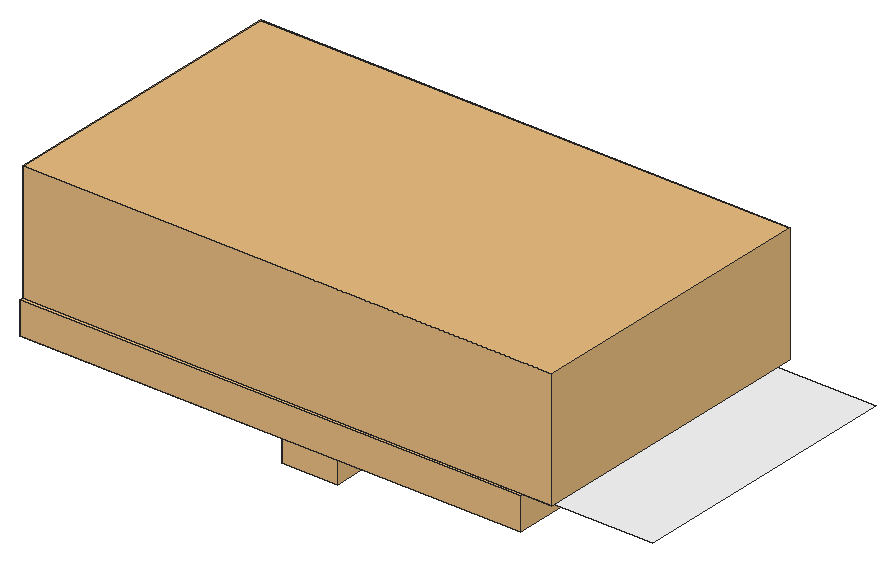
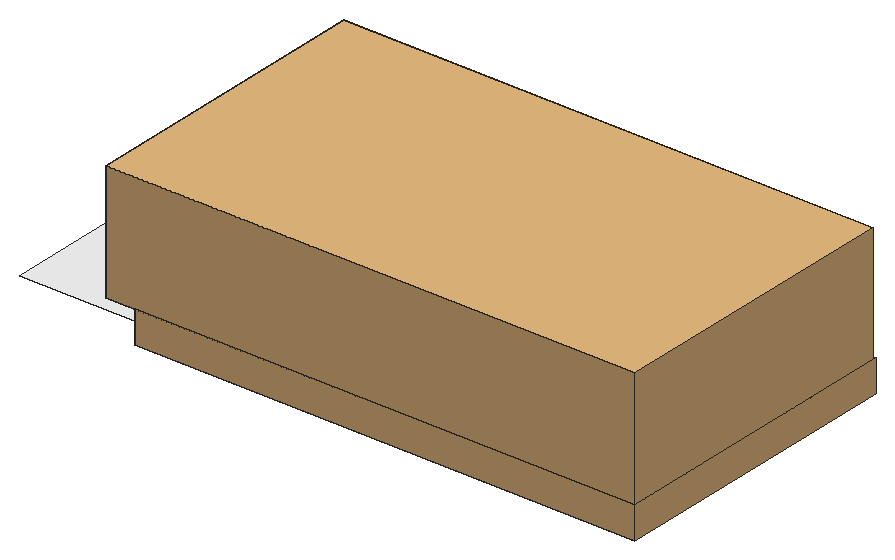
# SketchUp Ruby script. Lengths in inches.
U = 1.inch
M = Sketchup.active_model
def pt(a) = Geom::Point3d.new(a.map { |v| v * U })
def face(e, loops, mat)
  f = e.add_face(loops[0].map { |a| pt(a) })
  loops[1..].each { |l| e.add_face(l.map { |a| pt(a) }).erase! }
  f.material = f.back_material = mat if mat
  f
end
# faces: each face lists its corners as indices into pts; further lists are holes
def faces(e, pts, list, mat = nil) = list.each { |f| face(e, (f[0].is_a?(Array) ? f : [f]).map { |l| l.map { |i| pts[i] } }, mat) }
# xy, xz, yz: faces in a plane at the given z, y or x. An outline is a flat list of corners, or four numbers for a rectangle; further outlines are holes
def ring(l) = l.size == 4 ? [[l[0], l[1]], [l[2], l[1]], [l[2], l[3]], [l[0], l[3]]] : l.each_slice(2).to_a
def flat(e, list, mat, &to3) = list.each { |f| face(e, (f[0].is_a?(Array) ? f : [f]).map { |l| ring(l).map { |u, v| to3.(u, v) } }, mat) }
def xy(e, z, list, mat = nil) = flat(e, list, mat) { |x, y| [x, y, z] }
def xz(e, y, list, mat = nil) = flat(e, list, mat) { |x, z| [x, y, z] }
def yz(e, x, list, mat = nil) = flat(e, list, mat) { |y, z| [x, y, z] }
def lines(e, pts, list) = list.each { |a, b| e.add_line(pt(pts[a]), pt(pts[b])) }
# prism: a flat outline (further loops are holes) pulled along v
def prism(e, loops, v, mat = nil)
  f = face(e, loops, mat); d = Geom::Vector3d.new(v.map { |x| x * U })
  f.pushpull(f.normal.samedirection?(d) ? d.length : -d.length)
end
def box(e, o, s, mat = nil) = prism(e, [[o, [o[0] + s[0], o[1], o[2]], [o[0] + s[0], o[1] + s[1], o[2]], [o[0], o[1] + s[1], o[2]]]], [0, 0, s[2]], mat)
def at(x, y, z, deg = 0) = Geom::Transformation.translation(pt([x, y, z])) * Geom::Transformation.rotation(ORIGIN, Z_AXIS, deg.degrees)
def axes(o, x, y, z) = Geom::Transformation.new([*x, 0, *y, 0, *z, 0, *pt(o).to_a, 1])
def part(name) = M.definitions.add(name)
# library, detail: a bought-in or finely detailed component or shape, given as its bounding box
def library(name, o, s) = part(name).tap { |d| box(d.entities, o, s) }
def detail(e, o, s) = box(e.add_group.entities, o, s)
def put(e, d, t, mat = nil) = e.add_instance(d, t).tap { |i| i.material = mat if mat }
def group(e, t, mat = nil) = e.add_group.tap { |g| g.transformation = t; g.material = mat if mat }.entities
root = M.entities
M.materials.add("1421 AP 8232 ELEGANT GREY").color = [96, 96, 96]
M.materials.add("[Metal Seamed]").color = [36, 36, 35]
M.materials.add("[Quartz Light Grey]").color = [251, 251, 252]
c1 = library("Group\#16",[0,0,0],[139.79,84,8.95])
c2 = library("5",[-6.25,-6.25,-13.16],[15.58,15.58,13.16])
c3 = library("Group\#18",[0,-2,0],[147.82,83,33.01])
xy(root,119.5,[[115.18,204,114.86,204.04,114.79,204.05,114.71,204.07,114.63,204.08,114.56,204.1,114.48,204.125,114.41,204.15,114.33,204.17,114.19,204.23,114.11,204.26,114.04,204.29,113.97,204.33,113.9,204.36,113.83,204.4,113.77,204.44,113.7,204.48,113.63,204.53,113.57,204.57,113.45,204.67,113.38,204.72,113.33,204.77,113.27,204.82,113.1,204.99,112.95,205.17,112.91,205.24,112.86,205.3,112.82,205.37,112.78,205.43,112.66,205.64,112.59,205.78,112.5625,205.85,112.53,205.92,112.51,206,112.48,206.07,112.46,206.15,112.4375,206.22,112.42,206.3,112.38,206.45,112.36,206.61,112.35,206.6875,112.34,206.76,112.34,206.84,112.33,206.92,112.33,207.08,112.34,207.16,112.34,207.24,112.35,207.3125,112.36,207.39,112.38,207.55,112.42,207.7,112.4375,207.78,112.46,207.85,112.48,207.93,112.51,208,112.53,208.08,112.5625,208.15,112.59,208.22,112.66,208.36,112.78,208.57,112.82,208.63,112.86,208.7,112.91,208.76,112.95,208.83,113.1,209.01,113.27,209.18,113.33,209.23,113.38,209.28,113.45,209.33,113.57,209.43,113.63,209.47,113.7,209.52,113.77,209.56,113.83,209.6,113.9,209.64,113.97,209.67,114.04,209.71,114.11,209.74,114.19,209.77,114.33,209.83,114.41,209.85,114.48,209.875,114.56,209.9,114.63,209.92,114.71,209.93,114.79,209.95,114.86,209.96,115.18,210,115.49,210,115.65,209.98,115.72,209.97,115.88,209.95,115.96,209.93,116.03,209.92,116.11,209.9,116.19,209.875,116.26,209.85,116.33,209.83,116.41,209.8,116.55,209.74,116.625,209.71,116.7,209.67,116.76,209.64,116.97,209.52,117.03,209.47,117.1,209.43,117.4,209.18,117.45,209.12,117.51,209.07,117.5625,209.01,117.61,208.95,117.71,208.83,117.76,208.76,117.81,208.7,117.85,208.63,117.89,208.57,118.01,208.36,118.13,208.08,118.16,208,118.1875,207.93,118.21,207.85,118.23,207.78,118.25,207.7,118.27,207.625,118.28,207.55,118.3,207.47,118.31,207.39,118.32,207.3125,118.32,207.24,118.33,207.16,118.33,206.84,118.32,206.76,118.32,206.6875,118.31,206.61,118.3,206.53,118.28,206.45,118.27,206.375,118.25,206.3,118.23,206.22,118.21,206.15,118.1875,206.07,118.16,206,118.13,205.92,118.01,205.64,117.89,205.43,117.85,205.37,117.81,205.3,117.76,205.24,117.71,205.17,117.61,205.05,117.5625,204.99,117.51,204.93,117.45,204.88,117.4,204.82,117.1,204.57,117.03,204.53,116.97,204.48,116.76,204.36,116.7,204.33,116.625,204.29,116.55,204.26,116.41,204.2,116.33,204.17,116.26,204.15,116.19,204.125,116.11,204.1,116.03,204.08,115.96,204.07,115.88,204.05,115.72,204.03,115.65,204.02,115.49,204]],"[Quartz Light Grey]")
xy(root,126,[[60,187,174,187,174,193,216,193,216,271,60,271]],"[Quartz Light Grey]")
xz(root,204,[[115.18,117,115.25,119.5],[115.25,117,115.33,119.5],[115.33,117,115.41,119.5],[115.41,117,115.49,119.5]],"[Quartz Light Grey]")
xz(root,210,[[115.18,117,115.25,119.5],[115.25,117,115.33,119.5],[115.33,117,115.41,119.5],[115.41,117,115.49,119.5]],"[Quartz Light Grey]")
yz(root,72,[[206.84,117,206.92,119.5],[206.92,117,207,119.5],[207,117,207.08,119.5],[207.08,117,207.16,119.5]],"[Quartz Light Grey]")
yz(root,112.33,[[206.92,117,207,119.5],[207,117,207.08,119.5]],"[Quartz Light Grey]")
yz(root,112.34,[[206.76,117,206.84,119.5],[207.16,117,207.24,119.5]],"[Quartz Light Grey]")
yz(root,118.32,[[206.6875,117,206.76,119.5],[207.24,117,207.3125,119.5]],"[Quartz Light Grey]")
yz(root,118.33,[[206.84,117,206.92,119.5],[206.92,117,207,119.5],[207,117,207.08,119.5],[207.08,117,207.16,119.5]],"[Quartz Light Grey]")
yz(root,158.67,[[206.84,117,206.92,119.5],[206.92,117,207,119.5],[207,117,207.08,119.5],[207.08,117,207.16,119.5]],"[Quartz Light Grey]")
yz(root,158.68,[[206.6875,117,206.76,119.5],[207.24,117,207.3125,119.5]],"[Quartz Light Grey]")
p = [[114.86,204.04,117],[114.79,204.05,117],[114.79,204.05,119.5],[114.86,204.04,119.5],[114.94,204.03,117],[114.94,204.03,119.5],
  [115.02,204.02,117],[115.02,204.02,119.5],[115.1,204.01,117],[115.1,204.01,119.5],[115.18,204,117],[115.18,204,119.5],
  [115.57,204.01,117],[115.49,204,117],[115.49,204,119.5],[115.57,204.01,119.5],[115.65,204.02,117],[115.65,204.02,119.5],
  [115.72,204.03,117],[115.72,204.03,119.5],[115.8,204.04,117],[115.8,204.04,119.5],[115.88,204.05,117],[115.88,204.05,119.5],
  [69.78,204.1,117],[69.7,204.08,117],[69.7,204.08,119.5],[69.78,204.1,119.5],[69.85,204.125,117],[69.85,204.125,119.5],
  [69.93,204.15,117],[69.93,204.15,119.5],[70,204.17,117],[70,204.17,119.5],[114.41,204.15,117],[114.33,204.17,117],
  [114.33,204.17,119.5],[114.41,204.15,119.5],[114.48,204.125,117],[114.48,204.125,119.5],[114.56,204.1,117],[114.56,204.1,119.5],
  [114.63,204.08,117],[114.63,204.08,119.5],[114.71,204.07,117],[114.71,204.07,119.5],[115.96,204.07,117],[115.96,204.07,119.5],
  [116.03,204.08,117],[116.03,204.08,119.5],[116.11,204.1,117],[116.11,204.1,119.5],[116.19,204.125,117],[116.19,204.125,119.5],
  [116.26,204.15,117],[116.26,204.15,119.5],[116.33,204.17,117],[116.33,204.17,119.5],[70.08,204.2,117],[70.08,204.2,119.5],
  [70.15,204.23,117],[70.15,204.23,119.5],[70.22,204.26,117],[70.22,204.26,119.5],[114.19,204.23,117],[114.11,204.26,117],
  [114.11,204.26,119.5],[114.19,204.23,119.5],[114.26,204.2,117],[114.26,204.2,119.5],[116.41,204.2,117],[116.41,204.2,119.5],
  [116.48,204.23,117],[116.48,204.23,119.5],[116.55,204.26,117],[116.55,204.26,119.5],[70.29,204.29,117],[70.29,204.29,119.5],
  [70.36,204.33,117],[70.36,204.33,119.5],[70.43,204.36,117],[70.43,204.36,119.5],[113.97,204.33,117],[113.9,204.36,117],
  [113.9,204.36,119.5],[113.97,204.33,119.5],[114.04,204.29,117],[114.04,204.29,119.5],[116.625,204.29,117],[116.625,204.29,119.5],
  [116.7,204.33,117],[116.7,204.33,119.5],[116.76,204.36,117],[116.76,204.36,119.5],[70.5,204.4,117],[70.5,204.4,119.5],
  [70.57,204.44,117],[70.57,204.44,119.5],[70.63,204.48,117],[70.63,204.48,119.5],[113.77,204.44,117],[113.7,204.48,117],
  [113.7,204.48,119.5],[113.77,204.44,119.5],[113.83,204.4,117],[113.83,204.4,119.5],[116.83,204.4,117],[116.83,204.4,119.5],
  [116.9,204.44,117],[116.9,204.44,119.5],[116.97,204.48,117],[116.97,204.48,119.5],[70.7,204.53,117],[70.7,204.53,119.5],
  [70.76,204.57,117],[70.76,204.57,119.5],[113.63,204.53,117],[113.57,204.57,117],[113.57,204.57,119.5],[113.63,204.53,119.5],
  [117.03,204.53,117],[117.03,204.53,119.5],[117.1,204.57,117],[117.1,204.57,119.5],[70.83,204.62,117],[70.83,204.62,119.5],
  [70.89,204.67,117],[70.89,204.67,119.5],[113.51,204.62,117],[113.45,204.67,117],[113.45,204.67,119.5],[113.51,204.62,119.5],
  [117.16,204.62,117],[117.16,204.62,119.5],[117.22,204.67,117],[117.22,204.67,119.5],[70.95,204.72,117],[70.95,204.72,119.5],
  [71.01,204.77,117],[71.01,204.77,119.5],[113.38,204.72,117],[113.33,204.77,117],[113.33,204.77,119.5],[113.38,204.72,119.5],
  [117.28,204.72,117],[117.28,204.72,119.5],[117.34,204.77,117],[117.34,204.77,119.5],[71.07,204.82,117],[71.07,204.82,119.5],
  [71.12,204.88,117],[71.12,204.88,119.5],[113.27,204.82,117],[113.21,204.88,117],[113.21,204.88,119.5],[113.27,204.82,119.5],
  [117.4,204.82,117],[117.4,204.82,119.5],[117.45,204.88,117],[117.45,204.88,119.5],[71.18,204.93,117],[71.18,204.93,119.5],
  [71.23,204.99,117],[71.23,204.99,119.5],[113.16,204.93,117],[113.1,204.99,117],[113.1,204.99,119.5],[113.16,204.93,119.5],
  [117.51,204.93,117],[117.51,204.93,119.5],[117.5625,204.99,117],[117.5625,204.99,119.5],[71.28,205.05,117],[71.28,205.05,119.5],
  [113.05,205.05,117],[113.05,205.05,119.5],[117.61,205.05,117],[117.61,205.05,119.5],[71.33,205.11,117],[71.33,205.11,119.5],
  [71.38,205.17,117],[71.38,205.17,119.5],[113,205.11,117],[112.95,205.17,117],[112.95,205.17,119.5],[113,205.11,119.5],
  [117.66,205.11,117],[117.66,205.11,119.5],[117.71,205.17,117],[117.71,205.17,119.5],[159.34,205.11,117],[159.29,205.17,117],
  [159.29,205.17,119.5],[159.34,205.11,119.5],[71.43,205.24,117],[71.43,205.24,119.5],[71.47,205.3,117],[71.47,205.3,119.5],
  [112.91,205.24,117],[112.86,205.3,117],[112.86,205.3,119.5],[112.91,205.24,119.5],[117.76,205.24,117],[117.76,205.24,119.5],
  [117.81,205.3,117],[117.81,205.3,119.5],[159.24,205.24,117],[159.19,205.3,117],[159.19,205.3,119.5],[159.24,205.24,119.5],
  [71.52,205.37,117],[71.52,205.37,119.5],[112.82,205.37,117],[112.82,205.37,119.5],[117.85,205.37,117],[117.85,205.37,119.5],
  [159.15,205.37,117],[159.15,205.37,119.5],[71.56,205.43,117],[71.56,205.43,119.5],[71.6,205.5,117],[71.6,205.5,119.5],
  [112.78,205.43,117],[112.74,205.5,117],[112.74,205.5,119.5],[112.78,205.43,119.5],[117.89,205.43,117],[117.89,205.43,119.5],
  [117.93,205.5,117],[117.93,205.5,119.5],[159.11,205.43,117],[159.07,205.5,117],[159.07,205.5,119.5],[159.11,205.43,119.5],
  [71.64,205.57,117],[71.64,205.57,119.5],[112.7,205.57,117],[112.7,205.57,119.5],[117.97,205.57,117],[117.97,205.57,119.5],
  [159.03,205.57,117],[159.03,205.57,119.5],[71.67,205.64,117],[71.67,205.64,119.5],[71.71,205.71,117],[71.71,205.71,119.5],
  [112.66,205.64,117],[112.625,205.71,117],[112.625,205.71,119.5],[112.66,205.64,119.5],[118.01,205.64,117],[118.01,205.64,119.5],
  [118.04,205.71,117],[118.04,205.71,119.5],[158.99,205.64,117],[158.96,205.71,117],[158.96,205.71,119.5],[158.99,205.64,119.5],
  [71.74,205.78,117],[71.74,205.78,119.5],[112.59,205.78,117],[112.59,205.78,119.5],[118.07,205.78,117],[118.07,205.78,119.5],
  [158.93,205.78,117],[158.93,205.78,119.5],[71.77,205.85,117],[71.77,205.85,119.5],[112.5625,205.85,117],[112.5625,205.85,119.5],
  [118.1,205.85,117],[118.1,205.85,119.5],[158.9,205.85,117],[158.9,205.85,119.5],[71.8,205.92,117],[71.8,205.92,119.5],
  [71.83,206,117],[71.83,206,119.5],[112.53,205.92,117],[112.51,206,117],[112.51,206,119.5],[112.53,205.92,119.5],
  [118.13,205.92,117],[118.13,205.92,119.5],[118.16,206,117],[118.16,206,119.5],[158.87,205.92,117],[158.84,206,117],
  [158.84,206,119.5],[158.87,205.92,119.5],[71.85,206.07,117],[71.85,206.07,119.5],[112.48,206.07,117],[112.48,206.07,119.5],
  [118.1875,206.07,117],[118.1875,206.07,119.5],[158.8125,206.07,117],[158.8125,206.07,119.5],[71.875,206.15,117],[71.875,206.15,119.5],
  [71.9,206.22,117],[71.9,206.22,119.5],[112.46,206.15,117],[112.4375,206.22,117],[112.4375,206.22,119.5],[112.46,206.15,119.5],
  [118.21,206.15,117],[118.21,206.15,119.5],[118.23,206.22,117],[118.23,206.22,119.5],[158.79,206.15,117],[158.77,206.22,117],
  [158.77,206.22,119.5],[158.79,206.15,119.5],[71.92,206.3,117],[71.92,206.3,119.5],[112.42,206.3,117],[112.42,206.3,119.5],
  [118.25,206.3,117],[118.25,206.3,119.5],[158.75,206.3,117],[158.75,206.3,119.5],[71.93,206.375,117],[71.93,206.375,119.5],
  [112.4,206.375,117],[112.4,206.375,119.5],[118.27,206.375,117],[118.27,206.375,119.5],[158.73,206.375,117],[158.73,206.375,119.5],
  [71.95,206.45,117],[71.95,206.45,119.5],[112.38,206.45,117],[112.38,206.45,119.5],[118.28,206.45,117],[118.28,206.45,119.5],
  [158.72,206.45,117],[158.72,206.45,119.5],[71.96,206.53,117],[71.96,206.53,119.5],[71.97,206.61,117],[71.97,206.61,119.5],
  [112.37,206.53,117],[112.36,206.61,117],[112.36,206.61,119.5],[112.37,206.53,119.5],[118.3,206.53,117],[118.3,206.53,119.5],
  [118.31,206.61,117],[118.31,206.61,119.5],[158.7,206.53,117],[158.69,206.61,117],[158.69,206.61,119.5],[158.7,206.53,119.5],
  [71.98,206.6875,117],[71.98,206.6875,119.5],[112.35,206.6875,117],[112.35,206.6875,119.5],[118.32,206.6875,117],[118.32,206.6875,119.5],
  [158.68,206.6875,117],[158.68,206.6875,119.5],[71.99,206.76,117],[71.99,206.76,119.5],[112.34,206.76,117],[112.34,206.76,119.5],
  [72,206.84,117],[72,206.84,119.5],[112.34,206.84,117],[112.33,206.92,117],[112.33,206.92,119.5],[112.34,206.84,119.5],
  [118.33,206.84,117],[118.32,206.76,117],[118.32,206.76,119.5],[118.33,206.84,119.5],[158.68,206.76,117],[158.67,206.84,117],
  [158.67,206.84,119.5],[158.68,206.76,119.5],[112.33,207.08,117],[112.34,207.16,117],[112.34,207.16,119.5],[112.33,207.08,119.5],
  [71.98,207.3125,117],[71.99,207.24,117],[71.99,207.24,119.5],[71.98,207.3125,119.5],[72,207.16,117],[72,207.16,119.5],
  [112.34,207.24,117],[112.35,207.3125,117],[112.35,207.3125,119.5],[112.34,207.24,119.5],[118.32,207.24,117],[118.33,207.16,117],
  [118.33,207.16,119.5],[118.32,207.24,119.5],[158.67,207.16,117],[158.68,207.24,117],[158.68,207.24,119.5],[158.67,207.16,119.5],
  [71.97,207.39,117],[71.97,207.39,119.5],[112.36,207.39,117],[112.36,207.39,119.5],[118.31,207.39,117],[118.32,207.3125,117],
  [118.32,207.3125,119.5],[118.31,207.39,119.5],[158.68,207.3125,117],[158.69,207.39,117],[158.69,207.39,119.5],[158.68,207.3125,119.5],
  [71.96,207.47,117],[71.96,207.47,119.5],[112.37,207.47,117],[112.37,207.47,119.5],[118.3,207.47,117],[118.3,207.47,119.5],
  [158.7,207.47,117],[158.7,207.47,119.5],[71.93,207.625,117],[71.95,207.55,117],[71.95,207.55,119.5],[71.93,207.625,119.5],
  [112.38,207.55,117],[112.38,207.55,119.5],[112.4,207.625,117],[112.4,207.625,119.5],[118.27,207.625,117],[118.28,207.55,117],
  [118.28,207.55,119.5],[118.27,207.625,119.5],[158.72,207.55,117],[158.72,207.55,119.5],[158.73,207.625,117],[158.73,207.625,119.5],
  [71.92,207.7,117],[71.92,207.7,119.5],[112.42,207.7,117],[112.42,207.7,119.5],[118.25,207.7,117],[118.25,207.7,119.5],
  [158.75,207.7,117],[158.75,207.7,119.5],[71.9,207.78,117],[71.9,207.78,119.5],[112.4375,207.78,117],[112.4375,207.78,119.5],
  [118.23,207.78,117],[118.23,207.78,119.5],[158.77,207.78,117],[158.77,207.78,119.5],[71.875,207.85,117],[71.875,207.85,119.5],
  [112.46,207.85,117],[112.46,207.85,119.5],[118.21,207.85,117],[118.21,207.85,119.5],[158.79,207.85,117],[158.79,207.85,119.5],
  [71.83,208,117],[71.85,207.93,117],[71.85,207.93,119.5],[71.83,208,119.5],[112.48,207.93,117],[112.48,207.93,119.5],
  [112.51,208,117],[112.51,208,119.5],[118.16,208,117],[118.1875,207.93,117],[118.1875,207.93,119.5],[118.16,208,119.5],
  [158.8125,207.93,117],[158.8125,207.93,119.5],[158.84,208,117],[158.84,208,119.5],[71.8,208.08,117],[71.8,208.08,119.5],
  [112.53,208.08,117],[112.53,208.08,119.5],[118.13,208.08,117],[118.13,208.08,119.5],[158.87,208.08,117],[158.87,208.08,119.5],
  [71.74,208.22,117],[71.77,208.15,117],[71.77,208.15,119.5],[71.74,208.22,119.5],[112.5625,208.15,117],[112.5625,208.15,119.5],
  [112.59,208.22,117],[112.59,208.22,119.5],[118.07,208.22,117],[118.1,208.15,117],[118.1,208.15,119.5],[118.07,208.22,119.5],
  [158.9,208.15,117],[158.9,208.15,119.5],[158.93,208.22,117],[158.93,208.22,119.5],[71.71,208.29,117],[71.71,208.29,119.5],
  [112.625,208.29,117],[112.625,208.29,119.5],[118.04,208.29,117],[118.04,208.29,119.5],[158.96,208.29,117],[158.96,208.29,119.5],
  [71.67,208.36,117],[71.67,208.36,119.5],[112.66,208.36,117],[112.66,208.36,119.5],[118.01,208.36,117],[118.01,208.36,119.5],
  [158.99,208.36,117],[158.99,208.36,119.5],[71.6,208.5,117],[71.64,208.43,117],[71.64,208.43,119.5],[71.6,208.5,119.5],
  [112.7,208.43,117],[112.7,208.43,119.5],[112.74,208.5,117],[112.74,208.5,119.5],[117.93,208.5,117],[117.97,208.43,117],
  [117.97,208.43,119.5],[117.93,208.5,119.5],[159.03,208.43,117],[159.03,208.43,119.5],[159.07,208.5,117],[159.07,208.5,119.5],
  [71.56,208.57,117],[71.56,208.57,119.5],[112.78,208.57,117],[112.78,208.57,119.5],[117.89,208.57,117],[117.89,208.57,119.5],
  [159.11,208.57,117],[159.11,208.57,119.5],[71.47,208.7,117],[71.52,208.63,117],[71.52,208.63,119.5],[71.47,208.7,119.5],
  [112.82,208.63,117],[112.82,208.63,119.5],[112.86,208.7,117],[112.86,208.7,119.5],[117.81,208.7,117],[117.85,208.63,117],
  [117.85,208.63,119.5],[117.81,208.7,119.5],[159.15,208.63,117],[159.15,208.63,119.5],[159.19,208.7,117],[159.19,208.7,119.5],
  [71.43,208.76,117],[71.43,208.76,119.5],[112.91,208.76,117],[112.91,208.76,119.5],[117.76,208.76,117],[117.76,208.76,119.5],
  [159.24,208.76,117],[159.24,208.76,119.5],[71.33,208.89,117],[71.38,208.83,117],[71.38,208.83,119.5],[71.33,208.89,119.5],
  [112.95,208.83,117],[112.95,208.83,119.5],[113,208.89,117],[113,208.89,119.5],[117.66,208.89,117],[117.71,208.83,117],
  [117.71,208.83,119.5],[117.66,208.89,119.5],[159.29,208.83,117],[159.29,208.83,119.5],[71.23,209.01,117],[71.28,208.95,117],
  [71.28,208.95,119.5],[71.23,209.01,119.5],[113.05,208.95,117],[113.05,208.95,119.5],[113.1,209.01,117],[113.1,209.01,119.5],
  [117.5625,209.01,117],[117.61,208.95,117],[117.61,208.95,119.5],[117.5625,209.01,119.5],[71.18,209.07,117],[71.18,209.07,119.5],
  [113.16,209.07,117],[113.16,209.07,119.5],[117.51,209.07,117],[117.51,209.07,119.5],[71.07,209.18,117],[71.12,209.12,117],
  [71.12,209.12,119.5],[71.07,209.18,119.5],[113.21,209.12,117],[113.21,209.12,119.5],[113.27,209.18,117],[113.27,209.18,119.5],
  [117.4,209.18,117],[117.45,209.12,117],[117.45,209.12,119.5],[117.4,209.18,119.5],[70.95,209.28,117],[71.01,209.23,117],
  [71.01,209.23,119.5],[70.95,209.28,119.5],[113.33,209.23,117],[113.33,209.23,119.5],[113.38,209.28,117],[113.38,209.28,119.5],
  [117.28,209.28,117],[117.34,209.23,117],[117.34,209.23,119.5],[117.28,209.28,119.5],[70.83,209.38,117],[70.89,209.33,117],
  [70.89,209.33,119.5],[70.83,209.38,119.5],[113.45,209.33,117],[113.45,209.33,119.5],[113.51,209.38,117],[113.51,209.38,119.5],
  [117.16,209.38,117],[117.22,209.33,117],[117.22,209.33,119.5],[117.16,209.38,119.5],[70.7,209.47,117],[70.76,209.43,117],
  [70.76,209.43,119.5],[70.7,209.47,119.5],[113.57,209.43,117],[113.57,209.43,119.5],[113.63,209.47,117],[113.63,209.47,119.5],
  [117.03,209.47,117],[117.1,209.43,117],[117.1,209.43,119.5],[117.03,209.47,119.5],[70.57,209.56,117],[70.63,209.52,117],
  [70.63,209.52,119.5],[70.57,209.56,119.5],[113.7,209.52,117],[113.7,209.52,119.5],[113.77,209.56,117],[113.77,209.56,119.5],
  [116.9,209.56,117],[116.97,209.52,117],[116.97,209.52,119.5],[116.9,209.56,119.5],[70.36,209.67,117],[70.43,209.64,117],
  [70.43,209.64,119.5],[70.36,209.67,119.5],[70.5,209.6,117],[70.5,209.6,119.5],[113.83,209.6,117],[113.83,209.6,119.5],
  [113.9,209.64,117],[113.9,209.64,119.5],[113.97,209.67,117],[113.97,209.67,119.5],[116.7,209.67,117],[116.76,209.64,117],
  [116.76,209.64,119.5],[116.7,209.67,119.5],[116.83,209.6,117],[116.83,209.6,119.5],[70.15,209.77,117],[70.22,209.74,117],
  [70.22,209.74,119.5],[70.15,209.77,119.5],[70.29,209.71,117],[70.29,209.71,119.5],[114.04,209.71,117],[114.04,209.71,119.5],
  [114.11,209.74,117],[114.11,209.74,119.5],[114.19,209.77,117],[114.19,209.77,119.5],[116.48,209.77,117],[116.55,209.74,117],
  [116.55,209.74,119.5],[116.48,209.77,119.5],[116.625,209.71,117],[116.625,209.71,119.5],[69.93,209.85,117],[70,209.83,117],
  [70,209.83,119.5],[69.93,209.85,119.5],[70.08,209.8,117],[70.08,209.8,119.5],[114.26,209.8,117],[114.26,209.8,119.5],
  [114.33,209.83,117],[114.33,209.83,119.5],[114.41,209.85,117],[114.41,209.85,119.5],[116.26,209.85,117],[116.33,209.83,117],
  [116.33,209.83,119.5],[116.26,209.85,119.5],[116.41,209.8,117],[116.41,209.8,119.5],[69.7,209.92,117],[69.78,209.9,117],
  [69.78,209.9,119.5],[69.7,209.92,119.5],[69.85,209.875,117],[69.85,209.875,119.5],[114.48,209.875,117],[114.48,209.875,119.5],
  [114.56,209.9,117],[114.56,209.9,119.5],[114.63,209.92,117],[114.63,209.92,119.5],[114.71,209.93,117],[114.71,209.93,119.5],
  [114.79,209.95,117],[114.79,209.95,119.5],[114.86,209.96,117],[114.86,209.96,119.5],[115.8,209.96,117],[115.88,209.95,117],
  [115.88,209.95,119.5],[115.8,209.96,119.5],[115.96,209.93,117],[115.96,209.93,119.5],[116.03,209.92,117],[116.03,209.92,119.5],
  [116.11,209.9,117],[116.11,209.9,119.5],[116.19,209.875,117],[116.19,209.875,119.5],[114.94,209.97,117],[114.94,209.97,119.5],
  [115.02,209.98,117],[115.02,209.98,119.5],[115.1,209.99,117],[115.1,209.99,119.5],[115.18,210,117],[115.18,210,119.5],
  [115.49,210,117],[115.57,209.99,117],[115.57,209.99,119.5],[115.49,210,119.5],[115.65,209.98,117],[115.65,209.98,119.5],
  [115.72,209.97,117],[115.72,209.97,119.5],[44.18,187,128.99],[183.94,187,128.99]]
faces(root,p,[[0,1,2,3],[4,0,3,5],[6,4,5,7],[8,6,7,9],[10,8,9,11],[12,13,14,15],[16,12,15,17],[18,16,17,19],
  [20,18,19,21],[22,20,21,23],[24,25,26,27],[28,24,27,29],[30,28,29,31],[32,30,31,33],[34,35,36,37],[38,34,37,39],
  [40,38,39,41],[42,40,41,43],[44,42,43,45],[1,44,45,2],[46,22,23,47],[48,46,47,49],[50,48,49,51],[52,50,51,53],
  [54,52,53,55],[56,54,55,57],[58,32,33,59],[60,58,59,61],[62,60,61,63],[64,65,66,67],[68,64,67,69],[35,68,69,36],
  [70,56,57,71],[72,70,71,73],[74,72,73,75],[76,62,63,77],[78,76,77,79],[80,78,79,81],[82,83,84,85],[86,82,85,87],
  [65,86,87,66],[88,74,75,89],[90,88,89,91],[92,90,91,93],[94,80,81,95],[96,94,95,97],[98,96,97,99],[100,101,102,103],
  [104,100,103,105],[83,104,105,84],[106,92,93,107],[108,106,107,109],[110,108,109,111],[112,98,99,113],[114,112,113,115],[116,117,118,119],
  [101,116,119,102],[120,110,111,121],[122,120,121,123],[124,114,115,125],[126,124,125,127],[128,129,130,131],[117,128,131,118],[132,122,123,133],
  [134,132,133,135],[136,126,127,137],[138,136,137,139],[140,141,142,143],[129,140,143,130],[144,134,135,145],[146,144,145,147],[148,138,139,149],
  [150,148,149,151],[152,153,154,155],[141,152,155,142],[156,146,147,157],[158,156,157,159],[160,150,151,161],[162,160,161,163],[164,165,166,167],
  [153,164,167,154],[168,158,159,169],[170,168,169,171],[172,162,163,173],[165,174,175,166],[176,170,171,177],[178,172,173,179],[180,178,179,181],
  [182,183,184,185],[174,182,185,175],[186,176,177,187],[188,186,187,189],[190,191,192,193],[194,180,181,195],[196,194,195,197],[198,199,200,201],
  [183,198,201,184],[202,188,189,203],[204,202,203,205],[206,207,208,209],[191,206,209,192],[210,196,197,211],[199,212,213,200],[214,204,205,215],
  [207,216,217,208],[218,210,211,219],[220,218,219,221],[222,223,224,225],[212,222,225,213],[226,214,215,227],[228,226,227,229],[230,231,232,233],
  [216,230,233,217],[234,220,221,235],[223,236,237,224],[238,228,229,239],[231,240,241,232],[242,234,235,243],[244,242,243,245],[246,247,248,249],
  [236,246,249,237],[250,238,239,251],[252,250,251,253],[254,255,256,257],[240,254,257,241],[258,244,245,259],[247,260,261,248],[262,252,253,263],
  [255,264,265,256],[266,258,259,267],[260,268,269,261],[270,262,263,271],[264,272,273,265],[274,266,267,275],[276,274,275,277],[278,279,280,281],
  [268,278,281,269],[282,270,271,283],[284,282,283,285],[286,287,288,289],[272,286,289,273],[290,276,277,291],[279,292,293,280],[294,284,285,295],
  [287,296,297,288],[298,290,291,299],[300,298,299,301],[302,303,304,305],[292,302,305,293],[306,294,295,307],[308,306,307,309],[310,311,312,313],
  [296,310,313,297],[314,300,301,315],[303,316,317,304],[318,308,309,319],[311,320,321,312],[322,314,315,323],[316,324,325,317],[326,318,319,327],
  [320,328,329,321],[330,322,323,331],[324,332,333,325],[334,326,327,335],[328,336,337,329],[338,330,331,339],[340,338,339,341],[342,343,344,345],
  [332,342,345,333],[346,334,335,347],[348,346,347,349],[350,351,352,353],[336,350,353,337],[354,340,341,355],[343,356,357,344],[358,348,349,359],
  [351,360,361,352],[362,354,355,363],[356,364,365,357],[366,362,363,367],[368,369,370,371],[372,373,374,375],[376,377,378,379],[380,381,382,383],
  [384,385,386,387],[385,388,389,386],[390,391,392,393],[394,395,396,397],[398,399,400,401],[402,384,387,403],[391,404,405,392],[406,407,408,409],
  [410,411,412,413],[414,402,403,415],[404,416,417,405],[418,406,409,419],[411,420,421,412],[422,423,424,425],[423,414,415,424],[416,426,427,417],
  [426,428,429,427],[430,431,432,433],[431,418,419,432],[420,434,435,421],[434,436,437,435],[438,422,425,439],[428,440,441,429],[442,430,433,443],
  [436,444,445,437],[446,438,439,447],[440,448,449,441],[450,442,443,451],[444,452,453,445],[454,446,447,455],[448,456,457,449],[458,450,451,459],
  [452,460,461,453],[462,463,464,465],[463,454,455,464],[456,466,467,457],[466,468,469,467],[470,471,472,473],[471,458,459,472],[460,474,475,461],
  [474,476,477,475],[478,462,465,479],[468,480,481,469],[482,470,473,483],[476,484,485,477],[486,487,488,489],[487,478,479,488],[480,490,491,481],
  [490,492,493,491],[494,495,496,497],[495,482,483,496],[484,498,499,485],[498,500,501,499],[502,486,489,503],[492,504,505,493],[506,494,497,507],
  [500,508,509,501],[510,502,503,511],[504,512,513,505],[514,506,507,515],[508,516,517,509],[518,519,520,521],[519,510,511,520],[512,522,523,513],
  [522,524,525,523],[526,527,528,529],[527,514,515,528],[516,530,531,517],[530,532,533,531],[534,518,521,535],[524,536,537,525],[538,526,529,539],
  [532,540,541,533],[542,543,544,545],[543,534,535,544],[536,546,547,537],[546,548,549,547],[550,551,552,553],[551,538,539,552],[540,554,555,541],
  [554,556,557,555],[558,542,545,559],[548,560,561,549],[562,550,553,563],[556,564,565,557],[566,567,568,569],[567,558,559,568],[560,570,571,561],
  [570,572,573,571],[574,575,576,577],[575,562,563,576],[564,578,579,565],[580,581,582,583],[581,566,569,582],[572,584,585,573],[584,586,587,585],
  [588,589,590,591],[589,574,577,590],[592,580,583,593],[586,594,595,587],[596,588,591,597],[598,599,600,601],[599,592,593,600],[594,602,603,595],
  [602,604,605,603],[606,607,608,609],[607,596,597,608],[610,611,612,613],[611,598,601,612],[604,614,615,605],[614,616,617,615],[618,619,620,621],
  [619,606,609,620],[622,623,624,625],[623,610,613,624],[616,626,627,617],[626,628,629,627],[630,631,632,633],[631,618,621,632],[634,635,636,637],
  [635,622,625,636],[628,638,639,629],[638,640,641,639],[642,643,644,645],[643,630,633,644],[646,647,648,649],[647,634,637,648],[640,650,651,641],
  [650,652,653,651],[654,655,656,657],[655,642,645,656],[658,659,660,661],[659,662,663,660],[662,646,649,663],[652,664,665,653],[664,666,667,665],
  [666,668,669,667],[670,671,672,673],[671,674,675,672],[674,654,657,675],[676,677,678,679],[677,680,681,678],[680,658,661,681],[668,682,683,669],
  [682,684,685,683],[684,686,687,685],[688,689,690,691],[689,692,693,690],[692,670,673,693],[694,695,696,697],[695,698,699,696],[698,676,679,699],
  [686,700,701,687],[700,702,703,701],[702,704,705,703],[706,707,708,709],[707,710,711,708],[710,688,691,711],[712,713,714,715],[713,716,717,714],
  [716,694,697,717],[704,718,719,705],[718,720,721,719],[720,722,723,721],[722,724,725,723],[724,726,727,725],[726,728,729,727],[730,731,732,733],
  [731,734,735,732],[734,736,737,735],[736,738,739,737],[738,740,741,739],[740,706,709,741],[728,742,743,729],[742,744,745,743],[744,746,747,745],
  [746,748,749,747],[750,751,752,753],[751,754,755,752],[754,756,757,755],[756,730,733,757]],"[Quartz Light Grey]")
lines(root,p,[[758,759]])
put(root,c1,at(44.18,187,120.04),"1421 AP 8232 ELEGANT GREY")
put(root,c2,at(113.8,205.47,118.25),"[Quartz Light Grey]")
put(root,c3,at(44.18,190,128.99),"[Metal Seamed]")
